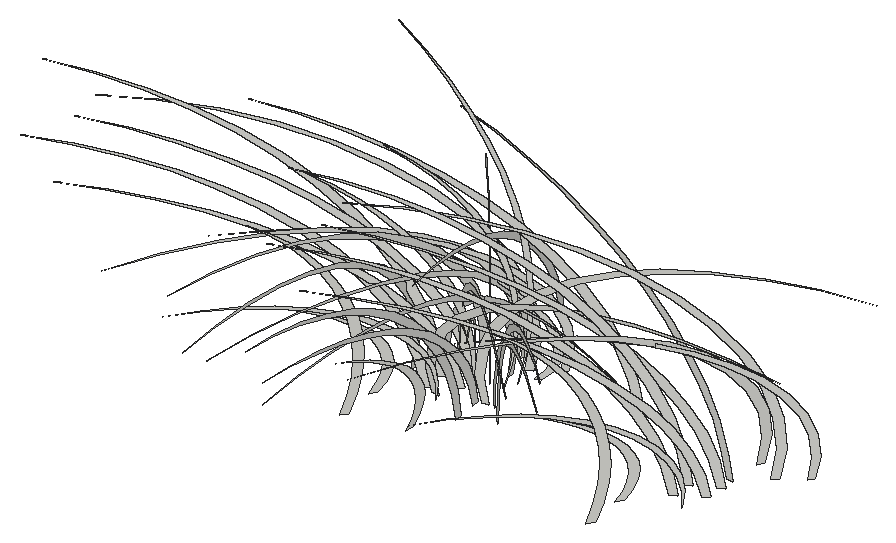
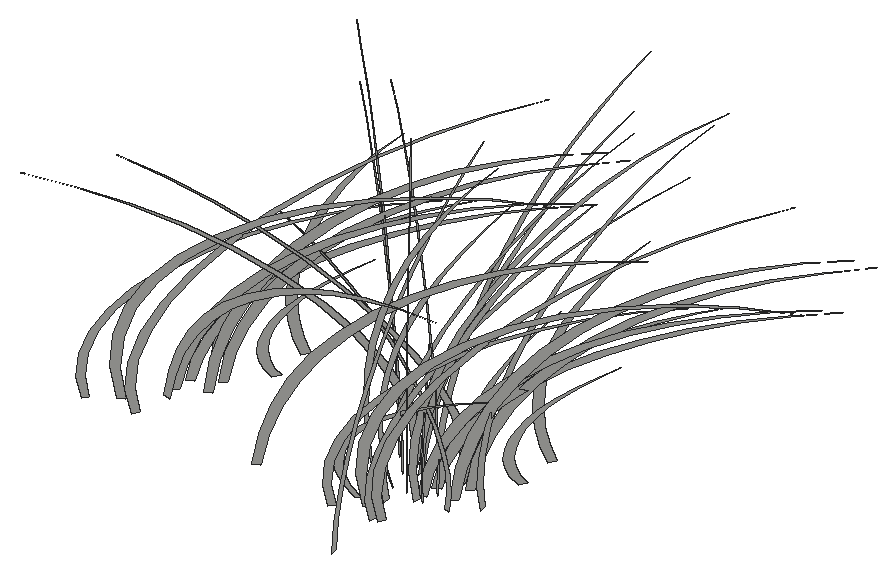
# SketchUp Ruby script. Lengths in inches.
U = 1.inch
M = Sketchup.active_model
def pt(a) = Geom::Point3d.new(a.map { |v| v * U })
def face(e, loops, mat)
  f = e.add_face(loops[0].map { |a| pt(a) })
  loops[1..].each { |l| e.add_face(l.map { |a| pt(a) }).erase! }
  f.material = f.back_material = mat if mat
  f
end
# faces: each face lists its corners as indices into pts; further lists are holes
def faces(e, pts, list, mat = nil) = list.each { |f| face(e, (f[0].is_a?(Array) ? f : [f]).map { |l| l.map { |i| pts[i] } }, mat) }
# xy, xz, yz: faces in a plane at the given z, y or x. An outline is a flat list of corners, or four numbers for a rectangle; further outlines are holes
def ring(l) = l.size == 4 ? [[l[0], l[1]], [l[2], l[1]], [l[2], l[3]], [l[0], l[3]]] : l.each_slice(2).to_a
def flat(e, list, mat, &to3) = list.each { |f| face(e, (f[0].is_a?(Array) ? f : [f]).map { |l| ring(l).map { |u, v| to3.(u, v) } }, mat) }
def xy(e, z, list, mat = nil) = flat(e, list, mat) { |x, y| [x, y, z] }
def xz(e, y, list, mat = nil) = flat(e, list, mat) { |x, z| [x, y, z] }
def yz(e, x, list, mat = nil) = flat(e, list, mat) { |y, z| [x, y, z] }
def lines(e, pts, list) = list.each { |a, b| e.add_line(pt(pts[a]), pt(pts[b])) }
# prism: a flat outline (further loops are holes) pulled along v
def prism(e, loops, v, mat = nil)
  f = face(e, loops, mat); d = Geom::Vector3d.new(v.map { |x| x * U })
  f.pushpull(f.normal.samedirection?(d) ? d.length : -d.length)
end
def box(e, o, s, mat = nil) = prism(e, [[o, [o[0] + s[0], o[1], o[2]], [o[0] + s[0], o[1] + s[1], o[2]], [o[0], o[1] + s[1], o[2]]]], [0, 0, s[2]], mat)
def at(x, y, z, deg = 0) = Geom::Transformation.translation(pt([x, y, z])) * Geom::Transformation.rotation(ORIGIN, Z_AXIS, deg.degrees)
def axes(o, x, y, z) = Geom::Transformation.new([*x, 0, *y, 0, *z, 0, *pt(o).to_a, 1])
def part(name) = M.definitions.add(name)
# library, detail: a bought-in or finely detailed component or shape, given as its bounding box
def library(name, o, s) = part(name).tap { |d| box(d.entities, o, s) }
def detail(e, o, s) = box(e.add_group.entities, o, s)
def put(e, d, t, mat = nil) = e.add_instance(d, t).tap { |i| i.material = mat if mat }
def group(e, t, mat = nil) = e.add_group.tap { |g| g.transformation = t; g.material = mat if mat }.entities
root = M.entities
g1 = group(root,at(366.56,267.27,0.02))
p = [[2.6,-20.61,15.34],[2.99,-23.72,15.75],[2.61,-20.71,15.26],[2.24,-17.8,14.58],[1.89,-15.03,13.72],[1.56,-12.42,12.69],
  [1.26,-10.01,11.5],[0.99,-7.82,10.16],[0.74,-5.88,8.7],[0.53,-4.21,7.11],[0.36,-2.83,5.43],[0.22,-1.74,3.67],
  [0.125,-0.98,1.86],[0.07,-0.54,0],[0,0,0],[0.05,-0.36,1.9],[0.14,-1.08,3.76],[0.27,-2.14,5.57],
  [0.45,-3.54,7.28],[0.66,-5.24,8.9],[0.91,-7.24,10.39],[1.2,-9.51,11.73],[1.51,-12.01,12.91],[1.85,-14.72,13.91],
  [2.22,-17.6,14.73]]
faces(g1,p,[[0,1,2,3,4,5,6,7,8,9,10,11,12,13,14,15,16,17,18,19,20,21,22,23,24]])
g2 = group(root,at(366.32,269.18,0.02))
p = [[2.6,-20.61,12.375],[2.99,-23.72,12.7],[2.61,-20.71,12.31],[2.24,-17.8,11.76],[1.89,-15.03,11.07],[1.56,-12.42,10.23],
  [1.26,-10.01,9.27],[0.99,-7.82,8.2],[0.74,-5.88,7.01],[0.53,-4.21,5.74],[0.36,-2.83,4.38],[0.22,-1.74,2.96],
  [0.125,-0.98,1.5],[0.07,-0.54,0],[0,0,0],[0.05,-0.36,1.53],[0.14,-1.08,3.03],[0.27,-2.14,4.49],
  [0.45,-3.54,5.875],[0.66,-5.24,7.18],[0.91,-7.24,8.375],[1.2,-9.51,9.46],[1.51,-12.01,10.41],[1.85,-14.72,11.22],
  [2.22,-17.6,11.88]]
faces(g2,p,[[0,1,2,3,4,5,6,7,8,9,10,11,12,13,14,15,16,17,18,19,20,21,22,23,24]])
g3 = group(root,at(360.78,270.68,0.02))
p = [[0.12,-0.92,0],[0.05,-0.41,0],[0,0,1.75],[0.02,-0.16,3.51],[0.11,-0.9,5.24],[0.27,-2.18,6.89],
  [0.5,-3.98,8.42],[0.79,-6.26,9.8],[1.13,-8.95,10.98],[1.51,-12,11.95],[1.93,-15.32,12.67],[2.37,-18.83,13.13],
  [2.83,-22.45,13.32],[3.28,-26.08,13.23],[2.84,-22.52,13.25],[2.39,-18.99,13],[1.96,-15.57,12.5],[1.56,-12.36,11.75],
  [1.19,-9.41,10.78],[0.86,-6.8,9.6],[0.58,-4.59,8.25],[0.36,-2.83,6.75],[0.2,-1.56,5.13],[0.1,-0.81,3.44],
  [0.07,-0.59,1.72]]
faces(g3,p,[[0,1,2,3,4,5,6,7,8,9,10,11,12,13,14,15,16,17,18,19,20,21,22,23,24]])
g4 = group(root,at(364.57,272.29,0.02))
p = [[-0.1,-0.92,0],[-0.05,-0.41,0],[0,0,2.0625],[-0.02,-0.17,4.13],[-0.1,-0.9,6.16],[-0.24,-2.1875,8.1],
  [-0.44,-3.99,9.91],[-0.69,-6.27,11.52],[-0.99,-8.97,12.92],[-1.33,-12.02,14.05],[-1.69,-15.34,14.9],[-2.08,-18.86,15.45],
  [-2.48,-22.49,15.67],[-2.88,-26.13,15.5625],[-2.49,-22.56,15.58],[-2.1,-19.02,15.29],[-1.72,-15.6,14.71],[-1.37,-12.38,13.83],
  [-1.04,-9.43,12.68],[-0.75,-6.81,11.3],[-0.51,-4.6,9.7],[-0.3125,-2.84,7.9375],[-0.17,-1.5625,6.04],[-0.09,-0.81,4.05],
  [-0.07,-0.59,2.02]]
faces(g4,p,[[0,1,2,3,4,5,6,7,8,9,10,11,12,13,14,15,16,17,18,19,20,21,22,23,24]])
g5 = group(root,at(364.57,272.29,0.02))
p = [[-0.1,-0.92,0],[-0.05,-0.41,0],[0,0,2.0625],[-0.02,-0.17,4.13],[-0.1,-0.9,6.16],[-0.24,-2.1875,8.1],
  [-0.44,-3.99,9.91],[-0.69,-6.27,11.52],[-0.99,-8.97,12.92],[-1.33,-12.02,14.05],[-1.69,-15.34,14.9],[-2.08,-18.86,15.45],
  [-2.48,-22.49,15.67],[-2.88,-26.13,15.5625],[-2.49,-22.56,15.58],[-2.1,-19.02,15.29],[-1.72,-15.6,14.71],[-1.37,-12.38,13.83],
  [-1.04,-9.43,12.68],[-0.75,-6.81,11.3],[-0.51,-4.6,9.7],[-0.3125,-2.84,7.9375],[-0.17,-1.5625,6.04],[-0.09,-0.81,4.05],
  [-0.07,-0.59,2.02]]
faces(g5,p,[[0,1,2,3,4,5,6,7,8,9,10,11,12,13,14,15,16,17,18,19,20,21,22,23,24]])
g6 = group(root,at(365.78,273.46,0.02))
p = [[0.125,-0.99,0],[0.06,-0.4375,0],[0,0,1.49],[0.02,-0.18,2.99],[0.12,-0.96,4.45],[0.3,-2.34,5.86],
  [0.54,-4.28,7.16],[0.85,-6.72,8.33],[1.21,-9.61,9.33],[1.62,-12.88,10.15],[2.07,-16.44,10.77],[2.55,-20.21,11.16],
  [3.03,-24.1,11.32],[3.53,-28,11.24],[3.04,-24.17,11.26],[2.57,-20.38,11.05],[2.11,-16.72,10.625],[1.67,-13.27,9.99],
  [1.27,-10.1,9.16],[0.92,-7.3,8.16],[0.62,-4.93,7.01],[0.38,-3.04,5.73],[0.21,-1.67,4.36],[0.11,-0.87,2.93],
  [0.08,-0.64,1.46]]
faces(g6,p,[[0,1,2,3,4,5,6,7,8,9,10,11,12,13,14,15,16,17,18,19,20,21,22,23,24]])
g7 = group(root,at(368.45,268.26,0.02))
p = [[14.61,-14.77,15.34],[16.8125,-17,15.75],[14.68,-14.84,15.26],[12.62,-12.76,14.58],[10.65,-10.77,13.72],[8.8,-8.9,12.69],
  [7.09,-7.17,11.5],[5.54,-5.61,10.16],[4.17,-4.22,8.7],[2.98,-3.02,7.11],[2,-2.02,5.43],[1.24,-1.25,3.67],
  [0.69,-0.7,1.86],[0.38,-0.38,0],[0,0,0],[0.26,-0.26,1.9],[0.77,-0.77,3.76],[1.52,-1.54,5.57],
  [2.51,-2.53,7.28],[3.72,-3.76,8.9],[5.13,-5.19,10.39],[6.74,-6.8125,11.73],[8.51,-8.61,12.91],[10.43,-10.55,13.91],
  [12.47,-12.61,14.73]]
faces(g7,p,[[0,1,2,3,4,5,6,7,8,9,10,11,12,13,14,15,16,17,18,19,20,21,22,23,24]])
g8 = group(root,at(383.5,266.89,0))
p = [[-9.23,-14.04,8.41],[-7.99,-12.15,8.36],[-6.77,-10.29,8.15],[-5.59,-8.5,7.8],[-4.48,-6.8125,7.32],[-3.46,-5.26,6.7],
  [-2.54,-3.86,5.97],[-1.75,-2.66,5.13],[-1.09,-1.67,4.2],[-0.59,-0.9,3.21],[-0.25,-0.39,2.16],[-0.08,-0.125,1.09],
  [-0.08,-0.125,0],[0,0,1.11],[-0.11,-0.16,2.21],[-0.4,-0.61,3.29],[-0.88,-1.34,4.32],[-1.53,-2.33,5.28],
  [-2.33,-3.55,6.14],[-3.27,-4.98,6.88],[-4.33,-6.59,7.5],[-5.48,-8.34,7.97],[-6.7,-10.19,8.28],[-7.96,-12.11,8.43]]
faces(g8,p,[[0,1,2,3,4,5,6,7,8,9,10,11,12,13,14,15,16,17,18,19,20,21,22,23]])
g9 = group(root,at(381.02,263.11,0))
p = [[-3.94,-6,13.62],[-3.22,-4.9,12.76],[-2.57,-3.91,11.81],[-2,-3.04,10.79],[-1.5,-2.28,9.7],[-1.09,-1.66,8.57],
  [-0.77,-1.17,7.38],[-0.54,-0.83,6.17],[-0.41,-0.62,4.93],[-0.37,-0.5625,3.6875],[-0.43,-0.65,2.44],[-0.58,-0.88,1.21],
  [-0.83,-1.26,0],[-0.51,-0.77,0],[-0.23,-0.36,1.22],[-0.0625,-0.1,2.48],[0,0,3.75],[-0.04,-0.07,5.02],
  [-0.19,-0.29,6.28],[-0.45,-0.68,7.51],[-0.8,-1.22,8.7],[-1.26,-1.91,9.84],[-1.81,-2.75,10.91],[-2.44,-3.71,11.9],
  [-3.16,-4.8,12.8125]]
faces(g9,p,[[0,1,2,3,4,5,6,7,8,9,10,11,12,13,14,15,16,17,18,19,20,21,22,23,24]])
g10 = group(root,at(364.33,267.96,0.02))
p = [[-9.23,-14.04,8.41],[-7.99,-12.15,8.36],[-6.77,-10.29,8.15],[-5.59,-8.5,7.8],[-4.48,-6.8125,7.32],[-3.46,-5.26,6.7],
  [-2.54,-3.86,5.97],[-1.75,-2.66,5.13],[-1.09,-1.67,4.2],[-0.59,-0.9,3.21],[-0.25,-0.39,2.16],[-0.08,-0.125,1.09],
  [-0.08,-0.125,0],[0,0,1.11],[-0.11,-0.16,2.21],[-0.4,-0.61,3.29],[-0.88,-1.34,4.32],[-1.53,-2.33,5.28],
  [-2.33,-3.55,6.14],[-3.27,-4.98,6.88],[-4.33,-6.59,7.5],[-5.48,-8.34,7.97],[-6.7,-10.19,8.28],[-7.96,-12.11,8.43]]
faces(g10,p,[[0,1,2,3,4,5,6,7,8,9,10,11,12,13,14,15,16,17,18,19,20,21,22,23]])
g11 = group(root,at(382.27,267.79,0))
p = [[-17.17,-11.7,15.34],[-19.76,-13.47,15.75],[-17.25,-11.76,15.26],[-14.83,-10.11,14.58],[-12.52,-8.53,13.72],[-10.35,-7.05,12.69],
  [-8.34,-5.68,11.5],[-6.52,-4.44,10.16],[-4.9,-3.34,8.7],[-3.51,-2.39,7.11],[-2.35,-1.6,5.43],[-1.45,-0.99,3.67],
  [-0.82,-0.56,1.86],[-0.45,-0.3,0],[0,0,0],[-0.3,-0.21,1.9],[-0.9,-0.61,3.76],[-1.78,-1.22,5.57],
  [-2.95,-2.01,7.28],[-4.37,-2.98,8.9],[-6.03,-4.11,10.39],[-7.92,-5.4,11.73],[-10,-6.82,12.91],[-12.26,-8.36,13.91],
  [-14.66,-9.99,14.73]]
faces(g11,p,[[0,1,2,3,4,5,6,7,8,9,10,11,12,13,14,15,16,17,18,19,20,21,22,23,24]])
g12 = group(root,at(367.09,269.64,0.02))
p = [[14.61,-14.77,12.375],[16.8125,-17,12.7],[14.68,-14.84,12.31],[12.62,-12.76,11.76],[10.65,-10.77,11.07],[8.8,-8.9,10.23],
  [7.09,-7.17,9.27],[5.54,-5.61,8.2],[4.17,-4.22,7.01],[2.98,-3.02,5.74],[2,-2.02,4.38],[1.24,-1.25,2.96],
  [0.69,-0.7,1.5],[0.38,-0.38,0],[0,0,0],[0.26,-0.26,1.53],[0.77,-0.77,3.03],[1.52,-1.54,4.49],
  [2.51,-2.53,5.875],[3.72,-3.76,7.18],[5.13,-5.19,8.375],[6.74,-6.8125,9.46],[8.51,-8.61,10.41],[10.43,-10.55,11.22],
  [12.47,-12.61,11.88]]
faces(g12,p,[[0,1,2,3,4,5,6,7,8,9,10,11,12,13,14,15,16,17,18,19,20,21,22,23,24]])
g13 = group(root,at(361.85,264.18,0.02))
p = [[-3.94,-6,13.62],[-3.22,-4.9,12.76],[-2.57,-3.91,11.81],[-2,-3.04,10.79],[-1.5,-2.28,9.7],[-1.09,-1.66,8.57],
  [-0.77,-1.17,7.38],[-0.54,-0.83,6.17],[-0.41,-0.62,4.93],[-0.37,-0.5625,3.6875],[-0.43,-0.65,2.44],[-0.58,-0.88,1.21],
  [-0.83,-1.26,0],[-0.51,-0.77,0],[-0.23,-0.36,1.22],[-0.0625,-0.1,2.48],[0,0,3.75],[-0.04,-0.07,5.02],
  [-0.19,-0.29,6.28],[-0.45,-0.68,7.51],[-0.8,-1.22,8.7],[-1.26,-1.91,9.84],[-1.81,-2.75,10.91],[-2.44,-3.71,11.9],
  [-3.16,-4.8,12.8125]]
faces(g13,p,[[0,1,2,3,4,5,6,7,8,9,10,11,12,13,14,15,16,17,18,19,20,21,22,23,24]])
g14 = group(root,at(383.98,274.38,0))
p = [[-0.37,-0.92,0],[-0.16,-0.41,0],[0,0,1.75],[-0.07,-0.17,3.51],[-0.36,-0.9,5.24],[-0.88,-2.19,6.89],
  [-1.61,-4,8.42],[-2.53,-6.28,9.8],[-3.61,-8.99,10.98],[-4.84,-12.04,11.95],[-6.18,-15.375,12.67],[-7.6,-18.9,13.13],
  [-9.06,-22.53,13.32],[-10.53,-26.18,13.23],[-9.09,-22.6,13.25],[-7.66,-19.06,13],[-6.29,-15.63,12.5],[-4.99,-12.41,11.75],
  [-3.8,-9.45,10.78],[-2.75,-6.83,9.6],[-1.85,-4.61,8.25],[-1.14,-2.84,6.75],[-0.63,-1.57,5.13],[-0.33,-0.8125,3.44],
  [-0.24,-0.59,1.72]]
faces(g14,p,[[0,1,2,3,4,5,6,7,8,9,10,11,12,13,14,15,16,17,18,19,20,21,22,23,24]])
g15 = group(root,at(363.57,270.77,0.02))
p = [[0.65,-0.66,0],[0.29,-0.29,0],[0,0,1.75],[0.12,-0.12,3.51],[0.64,-0.64,5.24],[1.55,-1.5625,6.89],
  [2.82,-2.86,8.42],[4.4375,-4.49,9.8],[6.35,-6.42,10.98],[8.5,-8.6,11.95],[10.85,-10.98,12.67],[13.34,-13.49,13.13],
  [15.91,-16.09,13.32],[18.48,-18.69,13.23],[15.96,-16.14,13.25],[13.45,-13.61,13],[11.04,-11.16,12.5],[8.76,-8.86,11.75],
  [6.67,-6.74,10.78],[4.82,-4.875,9.6],[3.25,-3.29,8.25],[2.01,-2.03,6.75],[1.11,-1.12,5.13],[0.57,-0.58,3.44],
  [0.42,-0.42,1.72]]
faces(g15,p,[[0,1,2,3,4,5,6,7,8,9,10,11,12,13,14,15,16,17,18,19,20,21,22,23,24]])
g16 = group(root,at(365.12,275.71,0.02))
p = [[-0.06,-0.99,0],[-0.03,-0.44,0],[0,0,1.49],[-0.01,-0.18,2.99],[-0.06,-0.97,4.45],[-0.14,-2.36,5.86],
  [-0.26,-4.3,7.16],[-0.4,-6.76,8.33],[-0.58,-9.67,9.33],[-0.77,-12.96,10.15],[-0.99,-16.54,10.77],[-1.22,-20.34,11.16],
  [-1.45,-24.24,11.32],[-1.68,-28.17,11.24],[-1.45,-24.32,11.26],[-1.23,-20.51,11.05],[-1.01,-16.82,10.625],[-0.8,-13.35,9.99],
  [-0.61,-10.16,9.16],[-0.4375,-7.35,8.16],[-0.3,-4.96,7.01],[-0.18,-3.06,5.73],[-0.1,-1.69,4.36],[-0.05,-0.87,2.93],
  [-0.04,-0.64,1.46]]
faces(g16,p,[[0,1,2,3,4,5,6,7,8,9,10,11,12,13,14,15,16,17,18,19,20,21,22,23,24]])
g17 = group(root,at(365.37,265.39,0.02))
p = [[-0.91,-7.12,6.7],[-0.75,-5.82,6.27],[-0.6,-4.64,5.81],[-0.46,-3.6,5.31],[-0.35,-2.71,4.77],[-0.25,-1.97,4.21],
  [-0.18,-1.39,3.63],[-0.125,-0.98,3.03],[-0.09,-0.74,2.43],[-0.09,-0.67,1.8125],[-0.1,-0.77,1.2],[-0.13,-1.05,0.59],
  [-0.19,-1.49,0],[-0.12,-0.92,0],[-0.05,-0.42,0.6],[-0.01,-0.11,1.22],[0,0,1.84],[-0.01,-0.08,2.47],
  [-0.04,-0.35,3.09],[-0.1,-0.81,3.69],[-0.1875,-1.45,4.28],[-0.29,-2.27,4.84],[-0.42,-3.26,5.37],[-0.57,-4.41,5.86],
  [-0.73,-5.7,6.3]]
faces(g17,p,[[0,1,2,3,4,5,6,7,8,9,10,11,12,13,14,15,16,17,18,19,20,21,22,23,24]])
g18 = group(root,at(363.1,268.85,0.02))
p = [[-17.17,-11.7,15.34],[-19.76,-13.47,15.75],[-17.25,-11.76,15.26],[-14.83,-10.11,14.58],[-12.52,-8.53,13.72],[-10.35,-7.05,12.69],
  [-8.34,-5.68,11.5],[-6.52,-4.44,10.16],[-4.9,-3.34,8.7],[-3.51,-2.39,7.11],[-2.35,-1.6,5.43],[-1.45,-0.99,3.67],
  [-0.82,-0.56,1.86],[-0.45,-0.3,0],[0,0,0],[-0.3,-0.21,1.9],[-0.9,-0.61,3.76],[-1.78,-1.22,5.57],
  [-2.95,-2.01,7.28],[-4.37,-2.98,8.9],[-6.03,-4.11,10.39],[-7.92,-5.4,11.73],[-10,-6.82,12.91],[-12.26,-8.36,13.91],
  [-14.66,-9.99,14.73]]
faces(g18,p,[[0,1,2,3,4,5,6,7,8,9,10,11,12,13,14,15,16,17,18,19,20,21,22,23,24]])
g19 = group(root,at(383.87,268.875,0))
p = [[-17.17,-11.7,12.375],[-19.76,-13.47,12.7],[-17.25,-11.76,12.31],[-14.83,-10.11,11.76],[-12.52,-8.53,11.07],[-10.35,-7.05,10.23],
  [-8.34,-5.68,9.27],[-6.52,-4.44,8.2],[-4.9,-3.34,7.01],[-3.51,-2.39,5.74],[-2.35,-1.6,4.38],[-1.45,-0.99,2.96],
  [-0.82,-0.56,1.5],[-0.45,-0.3,0],[0,0,0],[-0.3,-0.21,1.53],[-0.9,-0.61,3.03],[-1.78,-1.22,4.49],
  [-2.95,-2.01,5.875],[-4.37,-2.98,7.18],[-6.03,-4.11,8.375],[-7.92,-5.4,9.46],[-10,-6.82,10.41],[-12.26,-8.36,11.22],
  [-14.66,-9.99,11.88]]
faces(g19,p,[[0,1,2,3,4,5,6,7,8,9,10,11,12,13,14,15,16,17,18,19,20,21,22,23,24]])
g20 = group(root,at(364.8125,275.45,0.02))
p = [[-0.37,-0.92,0],[-0.16,-0.41,0],[0,0,1.75],[-0.07,-0.17,3.51],[-0.36,-0.9,5.24],[-0.88,-2.19,6.89],
  [-1.61,-4,8.42],[-2.53,-6.28,9.8],[-3.61,-8.99,10.98],[-4.84,-12.04,11.95],[-6.18,-15.375,12.67],[-7.6,-18.9,13.13],
  [-9.06,-22.53,13.32],[-10.53,-26.18,13.23],[-9.09,-22.6,13.25],[-7.66,-19.06,13],[-6.29,-15.63,12.5],[-4.99,-12.41,11.75],
  [-3.8,-9.45,10.78],[-2.75,-6.83,9.6],[-1.85,-4.61,8.25],[-1.14,-2.84,6.75],[-0.63,-1.57,5.13],[-0.33,-0.8125,3.44],
  [-0.24,-0.59,1.72]]
faces(g20,p,[[0,1,2,3,4,5,6,7,8,9,10,11,12,13,14,15,16,17,18,19,20,21,22,23,24]])
g21 = group(root,at(380.73,266.19,0))
p = [[-3.94,-6,6.7],[-3.22,-4.9,6.27],[-2.57,-3.91,5.81],[-2,-3.04,5.31],[-1.5,-2.28,4.77],[-1.09,-1.66,4.21],
  [-0.77,-1.17,3.63],[-0.54,-0.83,3.03],[-0.41,-0.62,2.43],[-0.37,-0.5625,1.8125],[-0.43,-0.65,1.2],[-0.58,-0.88,0.59],
  [-0.83,-1.26,0],[-0.51,-0.77,0],[-0.23,-0.36,0.6],[-0.0625,-0.1,1.22],[0,0,1.84],[-0.04,-0.07,2.47],
  [-0.19,-0.29,3.09],[-0.45,-0.68,3.69],[-0.8,-1.22,4.28],[-1.26,-1.91,4.84],[-1.81,-2.75,5.37],[-2.44,-3.71,5.86],
  [-3.16,-4.8,6.3]]
faces(g21,p,[[0,1,2,3,4,5,6,7,8,9,10,11,12,13,14,15,16,17,18,19,20,21,22,23,24]])
g22 = group(root,at(364.7,269.94,0.02))
p = [[-17.17,-11.7,12.375],[-19.76,-13.47,12.7],[-17.25,-11.76,12.31],[-14.83,-10.11,11.76],[-12.52,-8.53,11.07],[-10.35,-7.05,10.23],
  [-8.34,-5.68,9.27],[-6.52,-4.44,8.2],[-4.9,-3.34,7.01],[-3.51,-2.39,5.74],[-2.35,-1.6,4.38],[-1.45,-0.99,2.96],
  [-0.82,-0.56,1.5],[-0.45,-0.3,0],[0,0,0],[-0.3,-0.21,1.53],[-0.9,-0.61,3.03],[-1.78,-1.22,4.49],
  [-2.95,-2.01,5.875],[-4.37,-2.98,7.18],[-6.03,-4.11,8.375],[-7.92,-5.4,9.46],[-10,-6.82,10.41],[-12.26,-8.36,11.22],
  [-14.66,-9.99,11.88]]
faces(g22,p,[[0,1,2,3,4,5,6,7,8,9,10,11,12,13,14,15,16,17,18,19,20,21,22,23,24]])
g23 = group(root,at(382.23,269.28,0))
p = [[-18.45,-9.5625,18.05],[-21.23,-11,18.53],[-18.53,-9.61,17.95],[-15.93,-8.26,17.15],[-13.45,-6.97,16.14],[-11.12,-5.76,14.93],
  [-8.96,-4.64,13.53],[-7,-3.63,11.96],[-5.26,-2.73,10.23],[-3.77,-1.95,8.37],[-2.53,-1.3125,6.39],[-1.5625,-0.81,4.32],
  [-0.875,-0.45,2.18],[-0.48,-0.25,0],[0,0,0],[-0.32,-0.17,2.23],[-0.97,-0.5,4.43],[-1.92,-0.99,6.55],
  [-3.16,-1.64,8.57],[-4.69,-2.43,10.47],[-6.48,-3.36,12.22],[-8.51,-4.41,13.8],[-10.75,-5.57,15.1875],[-13.17,-6.83,16.37],
  [-15.75,-8.16,17.33]]
faces(g23,p,[[0,1,2,3,4,5,6,7,8,9,10,11,12,13,14,15,16,17,18,19,20,21,22,23,24]])
g24 = group(root,at(382.23,269.28,0))
p = [[-18.45,-9.5625,18.05],[-21.23,-11,18.53],[-18.53,-9.61,17.95],[-15.93,-8.26,17.15],[-13.45,-6.97,16.14],[-11.12,-5.76,14.93],
  [-8.96,-4.64,13.53],[-7,-3.63,11.96],[-5.26,-2.73,10.23],[-3.77,-1.95,8.37],[-2.53,-1.3125,6.39],[-1.5625,-0.81,4.32],
  [-0.875,-0.45,2.18],[-0.48,-0.25,0],[0,0,0],[-0.32,-0.17,2.23],[-0.97,-0.5,4.43],[-1.92,-0.99,6.55],
  [-3.16,-1.64,8.57],[-4.69,-2.43,10.47],[-6.48,-3.36,12.22],[-8.51,-4.41,13.8],[-10.75,-5.57,15.1875],[-13.17,-6.83,16.37],
  [-15.75,-8.16,17.33]]
faces(g24,p,[[0,1,2,3,4,5,6,7,8,9,10,11,12,13,14,15,16,17,18,19,20,21,22,23,24]])
g25 = group(root,at(361.56,267.26,0.02))
p = [[-3.94,-6,6.7],[-3.22,-4.9,6.27],[-2.57,-3.91,5.81],[-2,-3.04,5.31],[-1.5,-2.28,4.77],[-1.09,-1.66,4.21],
  [-0.77,-1.17,3.63],[-0.54,-0.83,3.03],[-0.41,-0.62,2.43],[-0.37,-0.5625,1.8125],[-0.43,-0.65,1.2],[-0.58,-0.88,0.59],
  [-0.83,-1.26,0],[-0.51,-0.77,0],[-0.23,-0.36,0.6],[-0.0625,-0.1,1.22],[0,0,1.84],[-0.04,-0.07,2.47],
  [-0.19,-0.29,3.09],[-0.45,-0.68,3.69],[-0.8,-1.22,4.28],[-1.26,-1.91,4.84],[-1.81,-2.75,5.37],[-2.44,-3.71,5.86],
  [-3.16,-4.8,6.3]]
faces(g25,p,[[0,1,2,3,4,5,6,7,8,9,10,11,12,13,14,15,16,17,18,19,20,21,22,23,24]])
g26 = group(root,at(383.94,270.17,0))
p = [[-18.45,-9.5625,14.56],[-21.23,-11,14.94],[-18.53,-9.61,14.48],[-15.93,-8.26,13.83],[-13.45,-6.97,13.02],[-11.12,-5.76,12.04],
  [-8.96,-4.64,10.91],[-7,-3.63,9.64],[-5.26,-2.73,8.25],[-3.77,-1.95,6.75],[-2.53,-1.3125,5.15],[-1.5625,-0.81,3.49],
  [-0.875,-0.45,1.76],[-0.48,-0.25,0],[0,0,0],[-0.32,-0.17,1.8],[-0.97,-0.5,3.57],[-1.92,-0.99,5.28],
  [-3.16,-1.64,6.91],[-4.69,-2.43,8.44],[-6.48,-3.36,9.85],[-8.51,-4.41,11.13],[-10.75,-5.57,12.25],[-13.17,-6.83,13.2],
  [-15.75,-8.16,13.97]]
faces(g26,p,[[0,1,2,3,4,5,6,7,8,9,10,11,12,13,14,15,16,17,18,19,20,21,22,23,24]])
g27 = group(root,at(383.94,270.17,0))
p = [[-18.45,-9.5625,14.56],[-21.23,-11,14.94],[-18.53,-9.61,14.48],[-15.93,-8.26,13.83],[-13.45,-6.97,13.02],[-11.12,-5.76,12.04],
  [-8.96,-4.64,10.91],[-7,-3.63,9.64],[-5.26,-2.73,8.25],[-3.77,-1.95,6.75],[-2.53,-1.3125,5.15],[-1.5625,-0.81,3.49],
  [-0.875,-0.45,1.76],[-0.48,-0.25,0],[0,0,0],[-0.32,-0.17,1.8],[-0.97,-0.5,3.57],[-1.92,-0.99,5.28],
  [-3.16,-1.64,6.91],[-4.69,-2.43,8.44],[-6.48,-3.36,9.85],[-8.51,-4.41,11.13],[-10.75,-5.57,12.25],[-13.17,-6.83,13.2],
  [-15.75,-8.16,13.97]]
faces(g27,p,[[0,1,2,3,4,5,6,7,8,9,10,11,12,13,14,15,16,17,18,19,20,21,22,23,24]])
g28 = group(root,at(363.06,270.35,0.02))
p = [[-18.45,-9.5625,18.05],[-21.23,-11,18.53],[-18.53,-9.61,17.95],[-15.93,-8.26,17.15],[-13.45,-6.97,16.14],[-11.12,-5.76,14.93],
  [-8.96,-4.64,13.53],[-7,-3.63,11.96],[-5.26,-2.73,10.23],[-3.77,-1.95,8.37],[-2.53,-1.3125,6.39],[-1.5625,-0.81,4.32],
  [-0.875,-0.45,2.18],[-0.48,-0.25,0],[0,0,0],[-0.32,-0.17,2.23],[-0.97,-0.5,4.43],[-1.92,-0.99,6.55],
  [-3.16,-1.64,8.57],[-4.69,-2.43,10.47],[-6.48,-3.36,12.22],[-8.51,-4.41,13.8],[-10.75,-5.57,15.1875],[-13.17,-6.83,16.37],
  [-15.75,-8.16,17.33]]
faces(g28,p,[[0,1,2,3,4,5,6,7,8,9,10,11,12,13,14,15,16,17,18,19,20,21,22,23,24]])
g29 = group(root,at(363.06,270.35,0.02))
p = [[-18.45,-9.5625,18.05],[-21.23,-11,18.53],[-18.53,-9.61,17.95],[-15.93,-8.26,17.15],[-13.45,-6.97,16.14],[-11.12,-5.76,14.93],
  [-8.96,-4.64,13.53],[-7,-3.63,11.96],[-5.26,-2.73,10.23],[-3.77,-1.95,8.37],[-2.53,-1.3125,6.39],[-1.5625,-0.81,4.32],
  [-0.875,-0.45,2.18],[-0.48,-0.25,0],[0,0,0],[-0.32,-0.17,2.23],[-0.97,-0.5,4.43],[-1.92,-0.99,6.55],
  [-3.16,-1.64,8.57],[-4.69,-2.43,10.47],[-6.48,-3.36,12.22],[-8.51,-4.41,13.8],[-10.75,-5.57,15.1875],[-13.17,-6.83,16.37],
  [-15.75,-8.16,17.33]]
faces(g29,p,[[0,1,2,3,4,5,6,7,8,9,10,11,12,13,14,15,16,17,18,19,20,21,22,23,24]])
g30 = group(root,at(365.58,269.86,0.02))
p = [[-5.83,-8.875,16.67],[-4.9,-7.46,15.44],[-4.05,-6.16,14.17],[-3.27,-4.98,12.86],[-2.58,-3.92,11.51],[-1.96,-2.98,10.14],
  [-1.43,-2.18,8.74],[-0.99,-1.5,7.31],[-0.63,-0.95,5.87],[-0.36,-0.54,4.42],[-0.17,-0.26,2.95],[-0.08,-0.12,1.48],
  [-0.08,-0.12,0],[0,0,1.48],[-0.03,-0.04,2.97],[-0.16,-0.24,4.45],[-0.4,-0.6,5.92],[-0.74,-1.12,7.37],
  [-1.18,-1.79,8.81],[-1.72,-2.61,10.21],[-2.36,-3.58,11.59],[-3.09,-4.7,12.93],[-3.92,-5.96,14.22],[-4.83,-7.35,15.47]]
faces(g30,p,[[0,1,2,3,4,5,6,7,8,9,10,11,12,13,14,15,16,17,18,19,20,21,22,23]])
g31 = group(root,at(364.77,271.23,0.02))
p = [[-18.45,-9.5625,14.56],[-21.23,-11,14.94],[-18.53,-9.61,14.48],[-15.93,-8.26,13.83],[-13.45,-6.97,13.02],[-11.12,-5.76,12.04],
  [-8.96,-4.64,10.91],[-7,-3.63,9.64],[-5.26,-2.73,8.25],[-3.77,-1.95,6.75],[-2.53,-1.3125,5.15],[-1.5625,-0.81,3.49],
  [-0.875,-0.45,1.76],[-0.48,-0.25,0],[0,0,0],[-0.32,-0.17,1.8],[-0.97,-0.5,3.57],[-1.92,-0.99,5.28],
  [-3.16,-1.64,6.91],[-4.69,-2.43,8.44],[-6.48,-3.36,9.85],[-8.51,-4.41,11.13],[-10.75,-5.57,12.25],[-13.17,-6.83,13.2],
  [-15.75,-8.16,13.97]]
faces(g31,p,[[0,1,2,3,4,5,6,7,8,9,10,11,12,13,14,15,16,17,18,19,20,21,22,23,24]])
g32 = group(root,at(364.77,271.23,0.02))
p = [[-18.45,-9.5625,14.56],[-21.23,-11,14.94],[-18.53,-9.61,14.48],[-15.93,-8.26,13.83],[-13.45,-6.97,13.02],[-11.12,-5.76,12.04],
  [-8.96,-4.64,10.91],[-7,-3.63,9.64],[-5.26,-2.73,8.25],[-3.77,-1.95,6.75],[-2.53,-1.3125,5.15],[-1.5625,-0.81,3.49],
  [-0.875,-0.45,1.76],[-0.48,-0.25,0],[0,0,0],[-0.32,-0.17,1.8],[-0.97,-0.5,3.57],[-1.92,-0.99,5.28],
  [-3.16,-1.64,6.91],[-4.69,-2.43,8.44],[-6.48,-3.36,9.85],[-8.51,-4.41,11.13],[-10.75,-5.57,12.25],[-13.17,-6.83,13.2],
  [-15.75,-8.16,13.97]]
faces(g32,p,[[0,1,2,3,4,5,6,7,8,9,10,11,12,13,14,15,16,17,18,19,20,21,22,23,24]])
g33 = group(root,at(387.49,274.53,0))
p = [[-0.5,-0.57,0],[-0.22,-0.25,0],[0,0,1.46],[-0.09,-0.1,2.93],[-0.49,-0.56,4.375],[-1.19,-1.35,5.75],
  [-2.17,-2.47,7.03],[-3.41,-3.89,8.18],[-4.88,-5.56,9.17],[-6.54,-7.45,9.98],[-8.36,-9.51,10.58],[-10.27,-11.69,10.97],
  [-12.24,-13.9375,11.125],[-14.23,-16.19,11.05],[-12.28,-13.98,11.0625],[-10.36,-11.79,10.86],[-8.5,-9.67,10.44],[-6.74,-7.67,9.82],
  [-5.13,-5.84,9.01],[-3.71,-4.22,8.02],[-2.51,-2.85,6.89],[-1.54,-1.76,5.64],[-0.85,-0.97,4.29],[-0.44,-0.5,2.88],
  [-0.32,-0.37,1.4375]]
faces(g33,p,[[0,1,2,3,4,5,6,7,8,9,10,11,12,13,14,15,16,17,18,19,20,21,22,23,24]])
g34 = group(root,at(386.07,273.19,0))
p = [[-0.82,-0.43,0],[-0.36,-0.1875,0],[0,0,2.0625],[-0.15,-0.08,4.13],[-0.8,-0.42,6.16],[-1.95,-1.01,8.1],
  [-3.57,-1.85,9.91],[-5.6,-2.9,11.52],[-8.01,-4.15,12.92],[-10.74,-5.57,14.05],[-13.71,-7.1,14.9],[-16.85,-8.73,15.45],
  [-20.09,-10.41,15.67],[-23.34,-12.1,15.5625],[-20.15,-10.44,15.58],[-16.99,-8.81,15.29],[-13.9375,-7.22,14.71],[-11.06,-5.73,13.83],
  [-8.42,-4.37,12.68],[-6.09,-3.16,11.3],[-4.11,-2.13,9.7],[-2.53,-1.3125,7.9375],[-1.4,-0.72,6.04],[-0.72,-0.375,4.05],
  [-0.53,-0.27,2.02]]
faces(g34,p,[[0,1,2,3,4,5,6,7,8,9,10,11,12,13,14,15,16,17,18,19,20,21,22,23,24]])
g35 = group(root,at(363.05,268.42,0.02))
p = [[0.99,-0.08,0],[0.44,-0.04,0],[0,0,1.49],[0.18,-0.01,2.99],[0.97,-0.08,4.45],[2.35,-0.19,5.86],
  [4.3,-0.35,7.16],[6.75,-0.55,8.33],[9.66,-0.78,9.33],[12.9375,-1.05,10.15],[16.52,-1.34,10.77],[20.31,-1.64,11.16],
  [24.21,-1.96,11.32],[28.13,-2.27,11.24],[24.28,-1.96,11.26],[20.48,-1.66,11.05],[16.8,-1.36,10.625],[13.33,-1.08,9.99],
  [10.15,-0.82,9.16],[7.34,-0.59,8.16],[4.95,-0.4,7.01],[3.05,-0.25,5.73],[1.68,-0.14,4.36],[0.87,-0.07,2.93],
  [0.64,-0.05,1.46]]
faces(g35,p,[[0,1,2,3,4,5,6,7,8,9,10,11,12,13,14,15,16,17,18,19,20,21,22,23,24]])
g36 = group(root,at(361.87,271.72,0.02))
p = [[0.69,-0.31,0],[0.31,-0.14,0],[0,0,1.24],[0.125,-0.06,2.49],[0.68,-0.3,3.72],[1.65,-0.73,4.89],
  [3.01,-1.34,5.98],[4.73,-2.11,6.95],[6.76,-3.01,7.8],[9.06,-4.04,8.48],[11.5625,-5.15,8.99],[14.21,-6.33,9.32],
  [16.94,-7.55,9.46],[19.6875,-8.77,9.39],[17,-7.58,9.4],[14.33,-6.39,9.23],[11.76,-5.24,8.875],[9.33,-4.16,8.35],
  [7.1,-3.17,7.65],[5.14,-2.29,6.82],[3.47,-1.55,5.86],[2.14,-0.95,4.79],[1.18,-0.52,3.64],[0.61,-0.27,2.45],
  [0.45,-0.2,1.22]]
faces(g36,p,[[0,1,2,3,4,5,6,7,8,9,10,11,12,13,14,15,16,17,18,19,20,21,22,23,24]])
g37 = group(root,at(368.32,275.6,0.02))
p = [[-0.5,-0.57,0],[-0.22,-0.25,0],[0,0,1.46],[-0.09,-0.1,2.93],[-0.49,-0.56,4.375],[-1.19,-1.35,5.75],
  [-2.17,-2.47,7.03],[-3.41,-3.89,8.18],[-4.88,-5.56,9.17],[-6.54,-7.45,9.98],[-8.36,-9.51,10.58],[-10.27,-11.69,10.97],
  [-12.24,-13.9375,11.125],[-14.23,-16.19,11.05],[-12.28,-13.98,11.0625],[-10.36,-11.79,10.86],[-8.5,-9.67,10.44],[-6.74,-7.67,9.82],
  [-5.13,-5.84,9.01],[-3.71,-4.22,8.02],[-2.51,-2.85,6.89],[-1.54,-1.76,5.64],[-0.85,-0.97,4.29],[-0.44,-0.5,2.88],
  [-0.32,-0.37,1.4375]]
faces(g37,p,[[0,1,2,3,4,5,6,7,8,9,10,11,12,13,14,15,16,17,18,19,20,21,22,23,24]])
g38 = group(root,at(368.32,275.6,0.02))
p = [[-0.5,-0.57,0],[-0.22,-0.25,0],[0,0,1.46],[-0.09,-0.1,2.93],[-0.49,-0.56,4.375],[-1.19,-1.35,5.75],
  [-2.17,-2.47,7.03],[-3.41,-3.89,8.18],[-4.88,-5.56,9.17],[-6.54,-7.45,9.98],[-8.36,-9.51,10.58],[-10.27,-11.69,10.97],
  [-12.24,-13.9375,11.125],[-14.23,-16.19,11.05],[-12.28,-13.98,11.0625],[-10.36,-11.79,10.86],[-8.5,-9.67,10.44],[-6.74,-7.67,9.82],
  [-5.13,-5.84,9.01],[-3.71,-4.22,8.02],[-2.51,-2.85,6.89],[-1.54,-1.76,5.64],[-0.85,-0.97,4.29],[-0.44,-0.5,2.88],
  [-0.32,-0.37,1.4375]]
faces(g38,p,[[0,1,2,3,4,5,6,7,8,9,10,11,12,13,14,15,16,17,18,19,20,21,22,23,24]])
g39 = group(root,at(366.9,274.26,0.02))
p = [[-0.82,-0.43,0],[-0.36,-0.1875,0],[0,0,2.0625],[-0.15,-0.08,4.13],[-0.8,-0.42,6.16],[-1.95,-1.01,8.1],
  [-3.57,-1.85,9.91],[-5.6,-2.9,11.52],[-8.01,-4.15,12.92],[-10.74,-5.57,14.05],[-13.71,-7.1,14.9],[-16.85,-8.73,15.45],
  [-20.09,-10.41,15.67],[-23.34,-12.1,15.5625],[-20.15,-10.44,15.58],[-16.99,-8.81,15.29],[-13.9375,-7.22,14.71],[-11.06,-5.73,13.83],
  [-8.42,-4.37,12.68],[-6.09,-3.16,11.3],[-4.11,-2.13,9.7],[-2.53,-1.3125,7.9375],[-1.4,-0.72,6.04],[-0.72,-0.375,4.05],
  [-0.53,-0.27,2.02]]
faces(g39,p,[[0,1,2,3,4,5,6,7,8,9,10,11,12,13,14,15,16,17,18,19,20,21,22,23,24]])
g40 = group(root,at(364.38,279.65,0.02))
p = [[6.07,-19.87,14.56],[6.99,-22.87,14.94],[6.1,-19.96,14.48],[5.25,-17.16,13.83],[4.43,-14.49,13.02],[3.66,-11.97,12.04],
  [2.95,-9.65,10.91],[2.31,-7.54,9.64],[1.73,-5.67,8.25],[1.24,-4.06,6.75],[0.83,-2.72,5.15],[0.51,-1.68,3.49],
  [0.29,-0.94,1.76],[0.16,-0.52,0],[0,0,0],[0.11,-0.35,1.8],[0.32,-1.04,3.57],[0.63,-2.07,5.28],
  [1.04,-3.41,6.91],[1.55,-5.05,8.44],[2.13,-6.98,9.85],[2.8,-9.16,11.13],[3.54,-11.58,12.25],[4.34,-14.1875,13.2],
  [5.1875,-16.96,13.97]]
faces(g40,p,[[0,1,2,3,4,5,6,7,8,9,10,11,12,13,14,15,16,17,18,19,20,21,22,23,24]])
g41 = group(root,at(367.04,272.08,0.02))
p = [[-0.52,-0.79,0],[-0.23,-0.35,1.51],[-0.06,-0.09,3.03],[0,0,4.56],[-0.06,-0.09,6.09],[-0.23,-0.35,7.61],
  [-0.52,-0.79,9.12],[-0.92,-1.39,10.61],[-1.43,-2.17,12.07],[-2.05,-3.12,13.5],[-2.78,-4.23,14.89],[-3.61,-5.49,16.24],
  [-4.54,-6.91,17.53],[-3.66,-5.57,16.21],[-2.88,-4.38,14.86],[-2.1875,-3.33,13.46],[-1.6,-2.43,12.03],[-1.1,-1.68,10.57],
  [-0.71,-1.08,9.08],[-0.42,-0.64,7.58],[-0.23,-0.35,6.07],[-0.15,-0.22,4.55],[-0.17,-0.25,3.03],[-0.29,-0.44,1.51]]
faces(g41,p,[[0,1,2,3,4,5,6,7,8,9,10,11,12,13,14,15,16,17,18,19,20,21,22,23]])
g42 = group(root,at(364.94,272.02,0.02))
p = [[0.57,-0.76,0],[0.25,-0.34,1.67],[0.0625,-0.09,3.36],[0,0,5.0625],[0.0625,-0.08,6.76],[0.25,-0.33,8.45],
  [0.5625,-0.75,10.12],[1,-1.34,11.77],[1.56,-2.08,13.4],[2.23,-2.99,14.98],[3.03,-4.05,16.53],[3.93,-5.26,18.02],
  [4.95,-6.62,19.46],[3.99,-5.34,18],[3.14,-4.2,16.49],[2.39,-3.19,14.9375],[1.74,-2.33,13.35],[1.2,-1.61,11.73],
  [0.77,-1.03,10.08],[0.46,-0.61,8.42],[0.25,-0.34,6.74],[0.16,-0.21,5.05],[0.18,-0.24,3.36],[0.32,-0.43,1.68]]
faces(g42,p,[[0,1,2,3,4,5,6,7,8,9,10,11,12,13,14,15,16,17,18,19,20,21,22,23]])
g43 = group(root,at(363.3125,272.67,0.02))
p = [[5.52,-7.72,6.7],[4.47,-6.25,6.27],[3.52,-4.92,5.81],[2.68,-3.75,5.31],[1.96,-2.74,4.77],[1.37,-1.91,4.21],
  [0.9,-1.26,3.63],[0.57,-0.79,3.03],[0.37,-0.52,2.43],[0.31,-0.44,1.8125],[0.4,-0.56,1.2],[0.62,-0.87,0.59],
  [0.98,-1.37,0],[0.74,-1.03,0],[0.33,-0.46,0.59],[0.07,-0.1,1.19],[-0.04,0.05,1.81],[0.01,-0.02,2.43],
  [0.21,-0.3,3.04],[0.5625,-0.79,3.65],[1.0625,-1.49,4.23],[1.7,-2.38,4.8],[2.48,-3.47,5.33],[3.38,-4.73,5.83],
  [4.4,-6.15,6.29]]
faces(g43,p,[[0,1,2,3,4,5,6,7,8,9,10,11,12,13,14,15,16,17,18,19,20,21,22,23,24]])
g44 = group(root,at(374.63,274.24,0.02))
p = [[-19.18,-7.98,16.73],[-22.08,-9.1875,17.17],[-19.27,-8.02,16.64],[-16.57,-6.9,15.9],[-13.98,-5.82,14.96],[-11.56,-4.8125,13.84],
  [-9.32,-3.88,12.54],[-7.28,-3.03,11.08],[-5.47,-2.28,9.48],[-3.92,-1.63,7.76],[-2.63,-1.09,5.92],[-1.625,-0.68,4.01],
  [-0.91,-0.38,2.02],[-0.5,-0.21,0],[0,0,0],[-0.34,-0.14,2.07],[-1.01,-0.42,4.1],[-1.99,-0.83,6.07],
  [-3.29,-1.37,7.94],[-4.88,-2.03,9.7],[-6.74,-2.81,11.33],[-8.85,-3.68,12.79],[-11.18,-4.65,14.08],[-13.7,-5.7,15.17],
  [-16.375,-6.82,16.0625]]
faces(g44,p,[[0,1,2,3,4,5,6,7,8,9,10,11,12,13,14,15,16,17,18,19,20,21,22,23,24]])
g45 = group(root,at(367.69,272.58,0.02))
p = [[-0.89,-0.32,0],[-0.4,-0.14,1.97],[-0.1,-0.04,3.96],[0,0,5.95],[-0.1,-0.03,7.95],[-0.39,-0.14,9.9375],
  [-0.89,-0.3125,11.91],[-1.57,-0.56,13.85],[-2.45,-0.87,15.76],[-3.52,-1.25,17.63],[-4.77,-1.6875,19.44],[-6.19,-2.19,21.2],
  [-7.79,-2.76,22.89],[-6.29,-2.23,21.17],[-4.94,-1.75,19.4],[-3.76,-1.33,17.58],[-2.74,-0.97,15.71],[-1.89,-0.67,13.8],
  [-1.22,-0.43,11.86],[-0.72,-0.25,9.9],[-0.4,-0.14,7.93],[-0.25,-0.09,5.94],[-0.29,-0.1,3.95],[-0.5,-0.18,1.97]]
faces(g45,p,[[0,1,2,3,4,5,6,7,8,9,10,11,12,13,14,15,16,17,18,19,20,21,22,23]])
g46 = group(root,at(366.14,269.13,0.02))
p = [[0.91,0.18,0],[0.4,0.08,0],[0,0,1.75],[0.16,0.03,3.51],[0.89,0.17,5.24],[2.16,0.42,6.89],
  [3.94,0.76,8.42],[6.19,1.2,9.8],[8.86,1.72,10.98],[11.87,2.3,11.95],[15.16,2.94,12.67],[18.63,3.61,13.13],
  [22.21,4.31,13.32],[25.81,5.01,13.23],[22.28,4.32,13.25],[18.79,3.64,13],[15.41,2.99,12.5],[12.23,2.37,11.75],
  [9.3125,1.81,10.78],[6.73,1.31,9.6],[4.54,0.88,8.25],[2.8,0.54,6.75],[1.54,0.3,5.13],[0.8,0.16,3.44],
  [0.59,0.11,1.72]]
faces(g46,p,[[0,1,2,3,4,5,6,7,8,9,10,11,12,13,14,15,16,17,18,19,20,21,22,23,24]])
g47 = group(root,at(368.79,273.94,0.02))
p = [[-9.01,-2.98,7.88],[-7.3,-2.41,7.38],[-5.75,-1.9,6.83],[-4.38,-1.45,6.24],[-3.2,-1.06,5.62],[-2.23,-0.74,4.96],
  [-1.47,-0.49,4.27],[-0.92,-0.31,3.57],[-0.61,-0.2,2.86],[-0.51,-0.17,2.13],[-0.65,-0.21,1.41],[-1.01,-0.33,0.7],
  [-1.6,-0.53,0],[-1.21,-0.4,0],[-0.54,-0.18,0.69],[-0.12,-0.04,1.4],[0.06,0.02,2.13],[-0.02,-0.01,2.85],
  [-0.35,-0.11,3.58],[-0.92,-0.3,4.29],[-1.73,-0.57,4.98],[-2.78,-0.92,5.64],[-4.05,-1.34,6.27],[-5.52,-1.82,6.86],
  [-7.18,-2.375,7.4]]
faces(g47,p,[[0,1,2,3,4,5,6,7,8,9,10,11,12,13,14,15,16,17,18,19,20,21,22,23,24]])
g48 = group(root,at(383.74,271.04,0))
p = [[-20.46,3.64,14.56],[-23.54,4.19,14.94],[-20.55,3.66,14.48],[-17.67,3.15,13.83],[-14.91,2.66,13.02],[-12.33,2.2,12.04],
  [-9.93,1.77,10.91],[-7.76,1.38,9.64],[-5.84,1.04,8.25],[-4.18,0.74,6.75],[-2.8,0.5,5.15],[-1.73,0.31,3.49],
  [-0.97,0.17,1.76],[-0.53,0.09,0],[0,0,0],[-0.36,0.0625,1.8],[-1.07,0.19,3.57],[-2.125,0.38,5.28],
  [-3.51,0.625,6.91],[-5.2,0.93,8.44],[-7.1875,1.28,9.85],[-9.43,1.68,11.13],[-11.92,2.125,12.25],[-14.61,2.6,13.2],
  [-17.46,3.11,13.97]]
faces(g48,p,[[0,1,2,3,4,5,6,7,8,9,10,11,12,13,14,15,16,17,18,19,20,21,22,23,24]])
